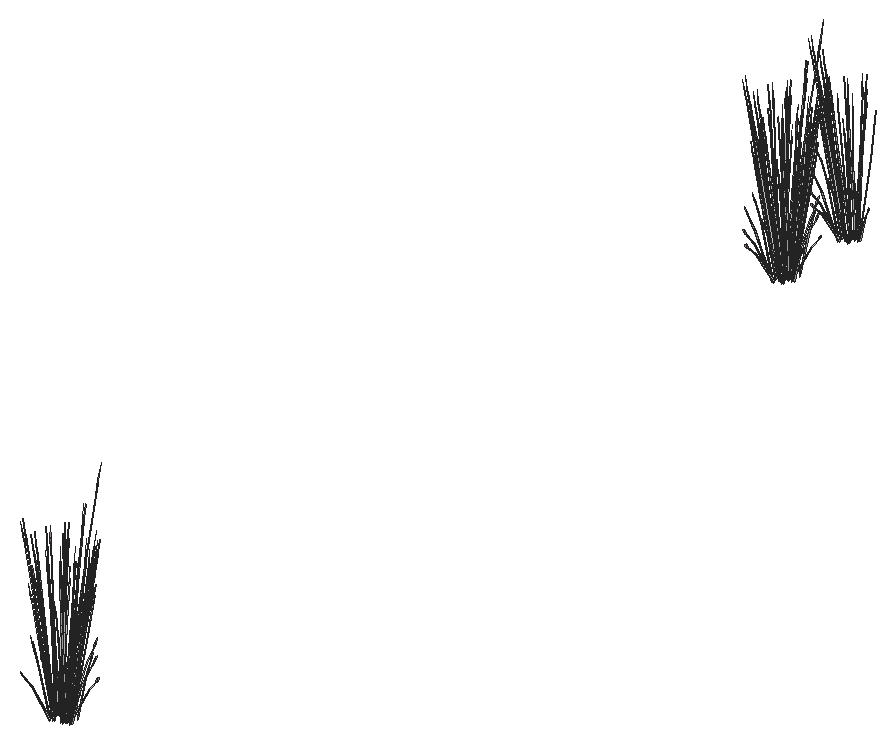
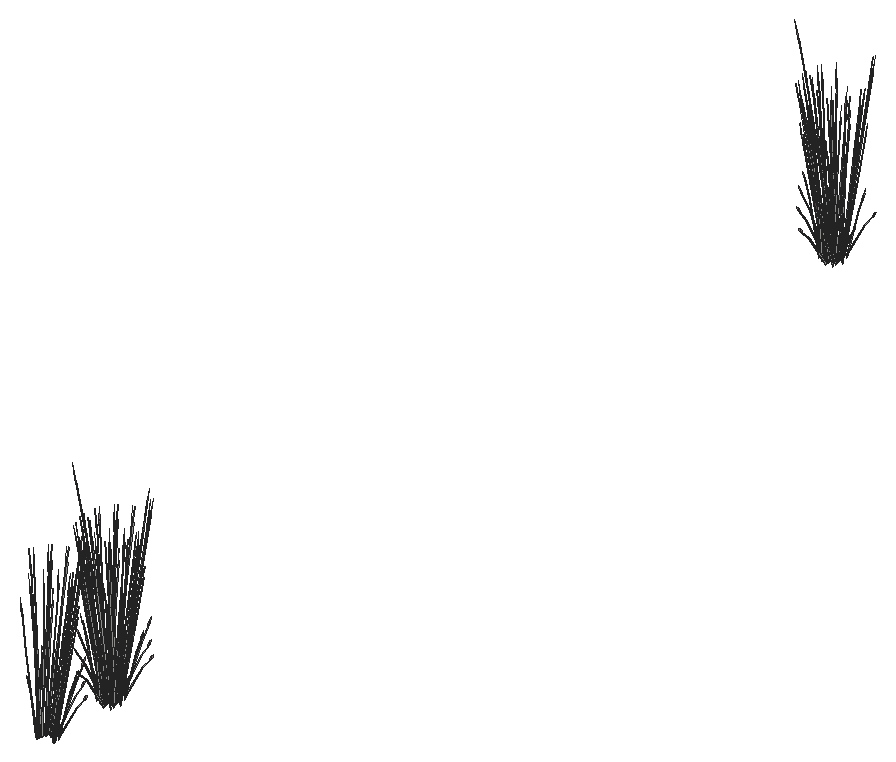
# SketchUp Ruby script. Lengths in inches.
U = 1.inch
M = Sketchup.active_model
def pt(a) = Geom::Point3d.new(a.map { |v| v * U })
def face(e, loops, mat)
  f = e.add_face(loops[0].map { |a| pt(a) })
  loops[1..].each { |l| e.add_face(l.map { |a| pt(a) }).erase! }
  f.material = f.back_material = mat if mat
  f
end
# faces: each face lists its corners as indices into pts; further lists are holes
def faces(e, pts, list, mat = nil) = list.each { |f| face(e, (f[0].is_a?(Array) ? f : [f]).map { |l| l.map { |i| pts[i] } }, mat) }
# xy, xz, yz: faces in a plane at the given z, y or x. An outline is a flat list of corners, or four numbers for a rectangle; further outlines are holes
def ring(l) = l.size == 4 ? [[l[0], l[1]], [l[2], l[1]], [l[2], l[3]], [l[0], l[3]]] : l.each_slice(2).to_a
def flat(e, list, mat, &to3) = list.each { |f| face(e, (f[0].is_a?(Array) ? f : [f]).map { |l| ring(l).map { |u, v| to3.(u, v) } }, mat) }
def xy(e, z, list, mat = nil) = flat(e, list, mat) { |x, y| [x, y, z] }
def xz(e, y, list, mat = nil) = flat(e, list, mat) { |x, z| [x, y, z] }
def yz(e, x, list, mat = nil) = flat(e, list, mat) { |y, z| [x, y, z] }
def lines(e, pts, list) = list.each { |a, b| e.add_line(pt(pts[a]), pt(pts[b])) }
# prism: a flat outline (further loops are holes) pulled along v
def prism(e, loops, v, mat = nil)
  f = face(e, loops, mat); d = Geom::Vector3d.new(v.map { |x| x * U })
  f.pushpull(f.normal.samedirection?(d) ? d.length : -d.length)
end
def box(e, o, s, mat = nil) = prism(e, [[o, [o[0] + s[0], o[1], o[2]], [o[0] + s[0], o[1] + s[1], o[2]], [o[0], o[1] + s[1], o[2]]]], [0, 0, s[2]], mat)
def at(x, y, z, deg = 0) = Geom::Transformation.translation(pt([x, y, z])) * Geom::Transformation.rotation(ORIGIN, Z_AXIS, deg.degrees)
def axes(o, x, y, z) = Geom::Transformation.new([*x, 0, *y, 0, *z, 0, *pt(o).to_a, 1])
def part(name) = M.definitions.add(name)
# library, detail: a bought-in or finely detailed component or shape, given as its bounding box
def library(name, o, s) = part(name).tap { |d| box(d.entities, o, s) }
def detail(e, o, s) = box(e.add_group.entities, o, s)
def put(e, d, t, mat = nil) = e.add_instance(d, t).tap { |i| i.material = mat if mat }
def group(e, t, mat = nil) = e.add_group.tap { |g| g.transformation = t; g.material = mat if mat }.entities
root = M.entities
M.materials.add("LightPink_Translucent").color = [144, 107, 117]
M.materials["LightPink_Translucent"].alpha = 0.75
c1 = part("blade")
p = [[2.15,0.21,22],[0,0.17,0],[0.09,0.45,0],[2.18,0.31,22],[2.29,0.31,22],[0.38,0.45,0],
  [2.48,0.24,33],[2.49,0.24,33],[2.48,0.22,33]]
faces(c1.entities,p,[[0,1,2,3],[4,5,2,3],[6,3,4,7],[8,0,3,6]])
c2 = part("seeds")
p = [[0.3,-0.1,1.38],[-0.01,-0.03,1.59],[-0.01,-0.03,0.03],[0.14,-0.07,-0.07],[0.29,-0.03,3],[0.15,0.01,3.11]]
faces(c2.entities,p,[[0,1,2,3],[1,0,4,5]],"LightPink_Translucent")
c3 = part("blade with seeds")
put(c3.entities,c1,at(0,0,0))
put(c3.entities,c2,axes([2.4,0.25,30.99],[1.5799,-0.05474,1.17369],[-0.12525,1.92788,0.29478],[-0.07173,-0.02425,1.56792]))
put(root,c3,axes([401.61,307.2,5.43],[-0.23555,0.44708,-0.13619],[-0.34112,-0.25757,-0.75594],[-0.11858,-0.12631,1.14864]))
put(root,c3,axes([403.22,307.69,4.73],[0.29004,0.02173,0.0643],[-0.00795,0.32812,0.50621],[0.03035,-0.12569,0.77189]))
put(root,c3,axes([403,307.91,5.05],[-0.23881,0.24554,0.35414],[-0.22606,-0.28036,-0.4572],[0.0344,-0.14245,0.87481]))
put(root,c3,axes([400.71,307.07,4.72],[-0.07594,-0.00329,1.74944],[-0.24177,0.32918,-0.27667],[-0.129,-0.06726,0.14031]))
put(root,c3,axes([403.58,308.71,5.03],[-0.32648,-0.25715,-0.1216],[0.18809,-0.3724,-0.67495],[0.09224,-0.12945,1.02557]))
put(root,c3,axes([401.59,307.57,5.05],[0.05451,0.37564,0.35414],[-0.31161,0.09919,-0.4572],[-0.0837,-0.10765,0.87481]))
put(root,c3,axes([400.65,307.8125,5.09],[0.29147,-0.34417,0.53763],[0.25138,0.3655,0.4433],[-0.13675,-0.06349,1.11249]))
put(root,c3,axes([404.38,308.6,4.71],[-0.0461,-0.00354,1.77383],[-0.19143,-0.37951,-0.16761],[0.07688,-0.12478,0.31391]))
put(root,c3,axes([400.78,307.8125,4.73],[0.01777,-0.35463,0.0643],[0.26836,0.00972,0.50621],[-0.1028,-0.03711,0.77189]))
put(root,c3,axes([403.42,308.67,5.05],[-0.30722,0.06665,0.35414],[-0.08112,-0.381,-0.4572],[0.08804,-0.10234,0.87481]))
put(root,c3,axes([403.7,308.61,4.73],[0.2423,0.19613,0.0643],[-0.14107,0.2793,0.50621],[0.07768,-0.0903,0.77189]))
put(root,c3,axes([403.63,308.53,4.73],[0.08753,0.42921,0.48003],[-0.34336,0.07449,0.3958],[0.1012,-0.10094,0.9933]))
put(root,c3,axes([404.55,309.05,4.72],[0.04898,-0.07104,1.74944],[-0.06269,-0.43574,-0.27667],[0.12289,-0.08262,0.14031]))
put(root,c3,axes([400.42,307.35,4.71],[0.02617,0.04654,1.77383],[-0.12614,0.41836,-0.16761],[-0.12775,0.00303,0.31391]))
put(root,c3,axes([400.97,308.08,5.05],[0.20082,0.29199,0.35414],[-0.2293,0.2764,-0.4572],[-0.1165,-0.04206,0.87481]))
put(root,c3,axes([400.91,307.89,5.03],[-0.0189,0.47427,-0.1216],[-0.35781,-0.01296,-0.67495],[-0.13781,-0.03295,1.02557]))
put(root,c3,axes([403.59,309.71,5.03],[-0.17758,-0.42229,-0.1216],[0.31518,-0.20752,-0.67495],[0.13282,-0.05572,1.02557]))
put(root,c3,axes([403.47,309.58,5.05],[-0.29332,-0.1301,0.35414],[0.08555,-0.37955,-0.4572],[0.11809,-0.0348,0.87481]))
put(root,c3,axes([400.4,308.89,4.73],[0.09971,-0.42522,0.48003],[0.32782,0.1454,0.3958],[-0.12892,0.02555,0.9933]))
put(root,c3,axes([400.37,308.78,4.73],[-0.12963,-0.31798,0.0643],[0.23638,-0.15564,0.50621],[-0.1042,0.03071,0.77189]))
put(root,c3,axes([403.73,309.7,4.73],[0.12963,0.31798,0.0643],[-0.23638,0.15564,0.50621],[0.1042,-0.03071,0.77189]))
put(root,c3,axes([403.71,309.59,4.73],[-0.09971,0.42522,0.48003],[-0.32782,-0.1454,0.3958],[0.12892,-0.02555,0.9933]))
put(root,c3,axes([400.64,308.9,5.05],[0.29332,0.1301,0.35414],[-0.08555,0.37955,-0.4572],[-0.11809,0.0348,0.87481]))
put(root,c3,axes([404.3,310.97,4.71],[-0.03191,-0.04083,1.77383],[0.06981,-0.43764,-0.16761],[0.12571,-0.02796,0.31391]))
put(root,c3,axes([400.14,309.19,4.72],[-0.05763,0.06055,1.74944],[0.0049,0.44239,-0.27667],[-0.13211,0.05753,0.14031]))
put(root,c3,axes([400.51,308.77,5.03],[0.17758,0.42229,-0.1216],[-0.31518,0.20752,-0.67495],[-0.13282,0.05572,1.02557]))
put(root,c3,axes([403.19,310.59,5.03],[0.0189,-0.47427,-0.1216],[0.35781,0.01296,-0.67495],[0.13781,0.03295,1.02557]))
put(root,c3,axes([403.14,310.4,5.05],[-0.20082,-0.29199,0.35414],[0.2293,-0.2764,-0.4572],[0.1165,0.04206,0.87481]))
put(root,c3,axes([403.5,310.3,4.72],[0.07571,-0.00789,1.74944],[0.20767,-0.36231,-0.27667],[0.13467,0.04783,0.14031]))
put(root,c3,axes([400.47,309.95,4.73],[-0.08753,-0.42921,0.48003],[0.34336,-0.07449,0.3958],[-0.1012,0.10094,0.9933]))
put(root,c3,axes([400.41,309.87,4.73],[-0.2423,-0.19613,0.0643],[0.14107,-0.2793,0.50621],[-0.07768,0.0903,0.77189]))
put(root,c3,axes([400.6875,309.81,5.05],[0.30722,-0.06665,0.35414],[0.08112,0.381,-0.4572],[-0.08804,0.10234,0.87481]))
put(root,c3,axes([399.5,309.64,4.71],[0.04504,0.01251,1.77383],[0.13934,0.41205,-0.16761],[-0.0922,0.10815,0.31391]))
put(root,c3,axes([403.32,310.67,4.73],[-0.01777,0.35463,0.0643],[-0.26836,-0.00972,0.50621],[0.1028,0.03711,0.77189]))
put(root,c3,axes([403.34,310.55,4.73],[-0.26024,0.30729,0.48003],[-0.22444,-0.32634,0.3958],[0.1221,0.05668,0.9933]))
put(root,c3,axes([399.99,310.89,5.65],[0.31145,0.12449,-0.06488],[-0.0958,0.38314,-0.29416],[-0.05094,0.05817,0.97024]))
put(root,c3,axes([402.52,310.91,5.05],[-0.05451,-0.37564,0.35414],[0.31161,-0.09919,-0.4572],[0.0837,0.10765,0.87481]))
put(root,c3,axes([402.72,308.75,4.47],[-0.30498,-0.24231,1.38283],[0.32203,-0.37727,0.59665],[0.0984,0.22736,1.33663]))
put(root,c3,axes([400.53,309.77,5.03],[0.32648,0.25715,-0.1216],[-0.18809,0.3724,-0.67495],[-0.09224,0.12945,1.02557]))
put(root,c3,axes([402.49,311.1,5.03],[0.21031,-0.39918,-0.1216],[0.30457,0.22997,-0.67495],[0.10587,0.11278,1.02557]))
put(root,c3,axes([401.1,310.57,5.05],[0.23881,-0.24554,0.35414],[0.22606,0.28036,-0.4572],[-0.0344,0.14245,0.87481]))
put(root,c3,axes([402.21,311.4375,4.71],[0.00104,-0.05646,1.77383],[0.30246,-0.2491,-0.16761],[0.10506,0.08891,0.31391]))
put(root,c3,axes([400.88,310.79,4.73],[-0.29004,-0.02173,0.0643],[0.00795,-0.32812,0.50621],[-0.03035,0.12569,0.77189]))
put(root,c3,axes([400.98,310.82,4.73],[-0.25132,-0.3182,0.48003],[0.2669,-0.27442,0.3958],[-0.04636,0.14929,0.9933]))
put(root,c3,axes([401.77,310.97,5.05],[0.1064,-0.35863,0.35414],[0.31043,0.1046,-0.4572],[0.02846,0.14439,0.87481]))
put(root,c3,axes([402.56,311.25,4.73],[-0.16041,0.29625,0.0643],[-0.22843,-0.17248,0.50621],[0.07385,0.09498,0.77189]))
put(root,c3,axes([402.1875,312.25,5.65],[0.2439,-0.26754,-0.06488],[0.22348,0.29302,-0.29416],[0.01573,0.08303,0.97024]))
put(root,c3,axes([402.63,311.17,4.73],[-0.35104,0.10702,0.48003],[-0.06092,-0.41983,0.3958],[0.08256,0.12373,0.9933]))
put(root,c3,axes([401.67,311.29,4.73],[-0.26007,0.1585,0.0643],[-0.12729,-0.28902,0.50621],[0.02512,0.1274,0.77189]))
put(root,c3,axes([400.15,310.84,4.72],[-0.00877,0.09229,1.74944],[0.24897,0.32105,-0.27667],[-0.06518,0.15182,0.14031]))
put(root,c3,axes([400.95,310.63,5.4],[0.3879,0.02311,-0.13498],[-0.0106,0.43749,-0.74919],[-0.02694,0.1685,1.13838]))
put(root,c3,axes([401.67,311.12,5.03],[0.34538,-0.21713,-0.1216],[0.16972,0.38536,-0.67495],[0.04557,0.16239,1.02557]))
put(root,c3,axes([401.77,311.26,5.0625],[-0.34777,-0.12192,0.53283],[0.11892,-0.40083,0.43934],[0.0209,0.15763,1.10256]))
put(root,c3,axes([400.125,311.79,4.71],[0.04004,-0.02816,1.77383],[0.33095,0.18728,-0.16761],[-0.00778,0.15594,0.31391]))
put(root,c3,axes([401.58,311.98,4.72],[0.04474,0.0751,1.74944],[0.36104,0.0295,-0.27667],[0.03631,0.16562,0.14031]))
put(root,c3,axes([401.89,516.79,4.72],[-0.05398,-0.06539,1.74944],[-0.36026,0.04145,-0.27667],[-0.0575,-0.15639,0.14031]))
put(root,c3,axes([403.51,517.59,4.72],[-0.00341,-0.09282,1.74944],[-0.28775,-0.26825,-0.27667],[0.04449,-0.16261,0.14031]))
put(root,c3,axes([403.43,517.25,4.71],[-0.03584,0.03562,1.77383],[-0.35118,-0.12018,-0.16761],[-0.01271,-0.15545,0.31391]))
put(root,c3,axes([401.52,516.57,4.71],[-0.00658,0.0559,1.77383],[-0.32474,0.20287,-0.16761],[-0.09556,-0.1037,0.31391]))
put(root,c3,axes([401.45,517.5625,5.09],[0.39316,-0.11987,0.53763],[0.06823,0.47021,0.4433],[-0.09247,-0.13858,1.11249]))
put(root,c3,axes([402.34,517.65,4.73],[0.34777,0.12192,0.48003],[-0.11892,0.40083,0.3958],[-0.0209,-0.15763,0.9933]))
put(root,c3,axes([402.4375,517.79,5.03],[-0.34538,0.21713,-0.1216],[-0.16972,-0.38536,-0.67495],[-0.04557,-0.16239,1.02557]))
put(root,c3,axes([403.15,518.28,5.03],[-0.3879,-0.02311,-0.1216],[0.0106,-0.43749,-0.67495],[0.02694,-0.1685,1.02557]))
put(root,c3,axes([402.43,517.62,4.73],[0.26007,-0.1585,0.0643],[0.12729,0.28902,0.50621],[-0.02512,-0.1274,0.77189]))
put(root,c3,axes([401.54,517.66,4.73],[0.16041,-0.29625,0.0643],[0.22843,0.17248,0.50621],[-0.07385,-0.09498,0.77189]))
put(root,c3,axes([402.33,517.95,5.05],[-0.1064,0.35863,0.35414],[-0.31043,-0.1046,-0.4572],[-0.02846,-0.14439,0.87481]))
put(root,c3,axes([403.125,518.1,4.73],[0.25132,0.3182,0.48003],[-0.2669,0.27442,0.3958],[0.04636,-0.14929,0.9933]))
put(root,c3,axes([401.61,517.63,5.43],[-0.23555,0.44708,-0.13619],[-0.34112,-0.25757,-0.75594],[-0.11858,-0.12631,1.14864]))
put(root,c3,axes([403.22,518.125,4.73],[0.29004,0.02173,0.0643],[-0.00795,0.32812,0.50621],[0.03035,-0.12569,0.77189]))
put(root,c3,axes([403,518.35,5.05],[-0.23881,0.24554,0.35414],[-0.22606,-0.28036,-0.4572],[0.0344,-0.14245,0.87481]))
put(root,c3,axes([400.71,517.51,4.72],[-0.07594,-0.00329,1.74944],[-0.24177,0.32918,-0.27667],[-0.129,-0.06726,0.14031]))
put(root,c3,axes([403.58,519.14,5.03],[-0.32648,-0.25715,-0.1216],[0.18809,-0.3724,-0.67495],[0.09224,-0.12945,1.02557]))
put(root,c3,axes([401.59,518.01,5.05],[0.05451,0.37564,0.35414],[-0.31161,0.09919,-0.4572],[-0.0837,-0.10765,0.87481]))
put(root,c3,axes([400.65,518.25,5.09],[0.29147,-0.34417,0.53763],[0.25138,0.3655,0.4433],[-0.13675,-0.06349,1.11249]))
put(root,c3,axes([404.38,519.03,4.71],[-0.0461,-0.00354,1.77383],[-0.19143,-0.37951,-0.16761],[0.07688,-0.12478,0.31391]))
put(root,c3,axes([400.78,518.25,4.73],[0.01777,-0.35463,0.0643],[0.26836,0.00972,0.50621],[-0.1028,-0.03711,0.77189]))
put(root,c3,axes([403.42,519.11,5.05],[-0.30722,0.06665,0.35414],[-0.08112,-0.381,-0.4572],[0.08804,-0.10234,0.87481]))
put(root,c3,axes([403.7,519.05,4.73],[0.2423,0.19613,0.0643],[-0.14107,0.2793,0.50621],[0.07768,-0.0903,0.77189]))
put(root,c3,axes([403.63,518.97,4.73],[0.08753,0.42921,0.48003],[-0.34336,0.07449,0.3958],[0.1012,-0.10094,0.9933]))
put(root,c3,axes([404.55,519.49,4.72],[0.04898,-0.07104,1.74944],[-0.06269,-0.43574,-0.27667],[0.12289,-0.08262,0.14031]))
put(root,c3,axes([400.42,517.78,4.71],[0.02617,0.04654,1.77383],[-0.12614,0.41836,-0.16761],[-0.12775,0.00303,0.31391]))
put(root,c3,axes([400.97,518.51,5.05],[0.20082,0.29199,0.35414],[-0.2293,0.2764,-0.4572],[-0.1165,-0.04206,0.87481]))
put(root,c3,axes([400.91,518.33,5.03],[-0.0189,0.47427,-0.1216],[-0.35781,-0.01296,-0.67495],[-0.13781,-0.03295,1.02557]))
put(root,c3,axes([403.59,520.15,5.03],[-0.17758,-0.42229,-0.1216],[0.31518,-0.20752,-0.67495],[0.13282,-0.05572,1.02557]))
put(root,c3,axes([403.47,520.02,5.05],[-0.29332,-0.1301,0.35414],[0.08555,-0.37955,-0.4572],[0.11809,-0.0348,0.87481]))
put(root,c3,axes([400.4,519.33,4.73],[0.09971,-0.42522,0.48003],[0.32782,0.1454,0.3958],[-0.12892,0.02555,0.9933]))
put(root,c3,axes([400.37,519.21,4.73],[-0.12963,-0.31798,0.0643],[0.23638,-0.15564,0.50621],[-0.1042,0.03071,0.77189]))
put(root,c3,axes([403.73,520.14,4.73],[0.12963,0.31798,0.0643],[-0.23638,0.15564,0.50621],[0.1042,-0.03071,0.77189]))
put(root,c3,axes([403.71,520.02,4.73],[-0.09971,0.42522,0.48003],[-0.32782,-0.1454,0.3958],[0.12892,-0.02555,0.9933]))
put(root,c3,axes([400.64,519.33,5.05],[0.29332,0.1301,0.35414],[-0.08555,0.37955,-0.4572],[-0.11809,0.0348,0.87481]))
put(root,c3,axes([404.3,521.4,4.71],[-0.03191,-0.04083,1.77383],[0.06981,-0.43764,-0.16761],[0.12571,-0.02796,0.31391]))
put(root,c3,axes([400.14,519.625,4.72],[-0.05763,0.06055,1.74944],[0.0049,0.44239,-0.27667],[-0.13211,0.05753,0.14031]))
put(root,c3,axes([400.51,519.2,5.03],[0.17758,0.42229,-0.1216],[-0.31518,0.20752,-0.67495],[-0.13282,0.05572,1.02557]))
put(root,c3,axes([403.19,521.02,5.03],[0.0189,-0.47427,-0.1216],[0.35781,0.01296,-0.67495],[0.13781,0.03295,1.02557]))
put(root,c3,axes([403.14,520.84,5.05],[-0.20082,-0.29199,0.35414],[0.2293,-0.2764,-0.4572],[0.1165,0.04206,0.87481]))
put(root,c3,axes([403.5,520.74,4.72],[0.07571,-0.00789,1.74944],[0.20767,-0.36231,-0.27667],[0.13467,0.04783,0.14031]))
put(root,c3,axes([400.47,520.39,4.73],[-0.08753,-0.42921,0.48003],[0.34336,-0.07449,0.3958],[-0.1012,0.10094,0.9933]))
put(root,c3,axes([400.41,520.3,4.73],[-0.2423,-0.19613,0.0643],[0.14107,-0.2793,0.50621],[-0.07768,0.0903,0.77189]))
put(root,c3,axes([400.6875,520.24,5.05],[0.30722,-0.06665,0.35414],[0.08112,0.381,-0.4572],[-0.08804,0.10234,0.87481]))
put(root,c3,axes([399.5,520.07,4.71],[0.04504,0.01251,1.77383],[0.13934,0.41205,-0.16761],[-0.0922,0.10815,0.31391]))
put(root,c3,axes([403.32,521.1,4.73],[-0.01777,0.35463,0.0643],[-0.26836,-0.00972,0.50621],[0.1028,0.03711,0.77189]))
put(root,c3,axes([403.34,520.99,4.73],[-0.26024,0.30729,0.48003],[-0.22444,-0.32634,0.3958],[0.1221,0.05668,0.9933]))
put(root,c3,axes([399.99,521.32,5.65],[0.31145,0.12449,-0.06488],[-0.0958,0.38314,-0.29416],[-0.05094,0.05817,0.97024]))
put(root,c3,axes([402.52,521.35,5.05],[-0.05451,-0.37564,0.35414],[0.31161,-0.09919,-0.4572],[0.0837,0.10765,0.87481]))
put(root,c3,axes([402.72,519.18,4.47],[-0.30498,-0.24231,1.38283],[0.32203,-0.37727,0.59665],[0.0984,0.22736,1.33663]))
put(root,c3,axes([400.53,520.21,5.03],[0.32648,0.25715,-0.1216],[-0.18809,0.3724,-0.67495],[-0.09224,0.12945,1.02557]))
put(root,c3,axes([402.49,521.54,5.03],[0.21031,-0.39918,-0.1216],[0.30457,0.22997,-0.67495],[0.10587,0.11278,1.02557]))
put(root,c3,axes([401.1,521,5.05],[0.23881,-0.24554,0.35414],[0.22606,0.28036,-0.4572],[-0.0344,0.14245,0.87481]))
put(root,c3,axes([402.21,521.87,4.71],[0.00104,-0.05646,1.77383],[0.30246,-0.2491,-0.16761],[0.10506,0.08891,0.31391]))
put(root,c3,axes([400.88,521.22,4.73],[-0.29004,-0.02173,0.0643],[0.00795,-0.32812,0.50621],[-0.03035,0.12569,0.77189]))
put(root,c3,axes([400.98,521.25,4.73],[-0.25132,-0.3182,0.48003],[0.2669,-0.27442,0.3958],[-0.04636,0.14929,0.9933]))
put(root,c3,axes([401.77,521.41,5.05],[0.1064,-0.35863,0.35414],[0.31043,0.1046,-0.4572],[0.02846,0.14439,0.87481]))
put(root,c3,axes([402.56,521.6875,4.73],[-0.16041,0.29625,0.0643],[-0.22843,-0.17248,0.50621],[0.07385,0.09498,0.77189]))
put(root,c3,axes([402.1875,522.68,5.65],[0.2439,-0.26754,-0.06488],[0.22348,0.29302,-0.29416],[0.01573,0.08303,0.97024]))
put(root,c3,axes([402.63,521.6,4.73],[-0.35104,0.10702,0.48003],[-0.06092,-0.41983,0.3958],[0.08256,0.12373,0.9933]))
put(root,c3,axes([401.67,521.73,4.73],[-0.26007,0.1585,0.0643],[-0.12729,-0.28902,0.50621],[0.02512,0.1274,0.77189]))
put(root,c3,axes([400.15,521.28,4.72],[-0.00877,0.09229,1.74944],[0.24897,0.32105,-0.27667],[-0.06518,0.15182,0.14031]))
put(root,c3,axes([400.95,521.07,5.4],[0.3879,0.02311,-0.13498],[-0.0106,0.43749,-0.74919],[-0.02694,0.1685,1.13838]))
put(root,c3,axes([401.67,521.56,5.03],[0.34538,-0.21713,-0.1216],[0.16972,0.38536,-0.67495],[0.04557,0.16239,1.02557]))
put(root,c3,axes([401.77,521.7,5.0625],[-0.34777,-0.12192,0.53283],[0.11892,-0.40083,0.43934],[0.0209,0.15763,1.10256]))
put(root,c3,axes([400.125,522.22,4.71],[0.04004,-0.02816,1.77383],[0.33095,0.18728,-0.16761],[-0.00778,0.15594,0.31391]))
put(root,c3,axes([401.58,522.42,4.72],[0.04474,0.0751,1.74944],[0.36104,0.0295,-0.27667],[0.03631,0.16562,0.14031]))
put(root,c3,axes([401.89,536.01,4.72],[-0.05398,-0.06539,1.74944],[-0.36026,0.04145,-0.27667],[-0.0575,-0.15639,0.14031]))
put(root,c3,axes([403.51,536.82,4.72],[-0.00341,-0.09282,1.74944],[-0.28775,-0.26825,-0.27667],[0.04449,-0.16261,0.14031]))
put(root,c3,axes([403.43,536.48,4.71],[-0.03584,0.03562,1.77383],[-0.35118,-0.12018,-0.16761],[-0.01271,-0.15545,0.31391]))
put(root,c3,axes([401.52,535.8,4.71],[-0.00658,0.0559,1.77383],[-0.32474,0.20287,-0.16761],[-0.09556,-0.1037,0.31391]))
put(root,c3,axes([401.45,536.79,5.09],[0.39316,-0.11987,0.53763],[0.06823,0.47021,0.4433],[-0.09247,-0.13858,1.11249]))
put(root,c3,axes([402.34,536.88,4.73],[0.34777,0.12192,0.48003],[-0.11892,0.40083,0.3958],[-0.0209,-0.15763,0.9933]))
put(root,c3,axes([402.4375,537.02,5.03],[-0.34538,0.21713,-0.1216],[-0.16972,-0.38536,-0.67495],[-0.04557,-0.16239,1.02557]))
put(root,c3,axes([403.15,537.51,5.03],[-0.3879,-0.02311,-0.1216],[0.0106,-0.43749,-0.67495],[0.02694,-0.1685,1.02557]))
put(root,c3,axes([402.43,536.85,4.73],[0.26007,-0.1585,0.0643],[0.12729,0.28902,0.50621],[-0.02512,-0.1274,0.77189]))
put(root,c3,axes([401.54,536.89,4.73],[0.16041,-0.29625,0.0643],[0.22843,0.17248,0.50621],[-0.07385,-0.09498,0.77189]))
put(root,c3,axes([402.33,537.17,5.05],[-0.1064,0.35863,0.35414],[-0.31043,-0.1046,-0.4572],[-0.02846,-0.14439,0.87481]))
put(root,c3,axes([403.125,537.33,4.73],[0.25132,0.3182,0.48003],[-0.2669,0.27442,0.3958],[0.04636,-0.14929,0.9933]))
put(root,c3,axes([401.61,536.86,5.43],[-0.23555,0.44708,-0.13619],[-0.34112,-0.25757,-0.75594],[-0.11858,-0.12631,1.14864]))
put(root,c3,axes([403.22,537.36,4.73],[0.29004,0.02173,0.0643],[-0.00795,0.32812,0.50621],[0.03035,-0.12569,0.77189]))
put(root,c3,axes([403,537.58,5.05],[-0.23881,0.24554,0.35414],[-0.22606,-0.28036,-0.4572],[0.0344,-0.14245,0.87481]))
put(root,c3,axes([400.71,536.73,4.72],[-0.07594,-0.00329,1.74944],[-0.24177,0.32918,-0.27667],[-0.129,-0.06726,0.14031]))
put(root,c3,axes([403.58,538.37,5.03],[-0.32648,-0.25715,-0.1216],[0.18809,-0.3724,-0.67495],[0.09224,-0.12945,1.02557]))
put(root,c3,axes([401.59,537.23,5.05],[0.05451,0.37564,0.35414],[-0.31161,0.09919,-0.4572],[-0.0837,-0.10765,0.87481]))
put(root,c3,axes([400.65,537.48,5.09],[0.29147,-0.34417,0.53763],[0.25138,0.3655,0.4433],[-0.13675,-0.06349,1.11249]))
put(root,c3,axes([404.38,538.26,4.71],[-0.0461,-0.00354,1.77383],[-0.19143,-0.37951,-0.16761],[0.07688,-0.12478,0.31391]))
put(root,c3,axes([400.78,537.48,4.73],[0.01777,-0.35463,0.0643],[0.26836,0.00972,0.50621],[-0.1028,-0.03711,0.77189]))
put(root,c3,axes([403.42,538.34,5.05],[-0.30722,0.06665,0.35414],[-0.08112,-0.381,-0.4572],[0.08804,-0.10234,0.87481]))
put(root,c3,axes([403.7,538.28,4.73],[0.2423,0.19613,0.0643],[-0.14107,0.2793,0.50621],[0.07768,-0.0903,0.77189]))
put(root,c3,axes([403.63,538.19,4.73],[0.08753,0.42921,0.48003],[-0.34336,0.07449,0.3958],[0.1012,-0.10094,0.9933]))
put(root,c3,axes([404.55,538.71,4.72],[0.04898,-0.07104,1.74944],[-0.06269,-0.43574,-0.27667],[0.12289,-0.08262,0.14031]))
put(root,c3,axes([400.42,537.01,4.71],[0.02617,0.04654,1.77383],[-0.12614,0.41836,-0.16761],[-0.12775,0.00303,0.31391]))
put(root,c3,axes([400.97,537.74,5.05],[0.20082,0.29199,0.35414],[-0.2293,0.2764,-0.4572],[-0.1165,-0.04206,0.87481]))
put(root,c3,axes([400.91,537.55,5.03],[-0.0189,0.47427,-0.1216],[-0.35781,-0.01296,-0.67495],[-0.13781,-0.03295,1.02557]))
put(root,c3,axes([403.59,539.375,5.03],[-0.17758,-0.42229,-0.1216],[0.31518,-0.20752,-0.67495],[0.13282,-0.05572,1.02557]))
put(root,c3,axes([403.47,539.25,5.05],[-0.29332,-0.1301,0.35414],[0.08555,-0.37955,-0.4572],[0.11809,-0.0348,0.87481]))
put(root,c3,axes([400.4,538.55,4.73],[0.09971,-0.42522,0.48003],[0.32782,0.1454,0.3958],[-0.12892,0.02555,0.9933]))
put(root,c3,axes([400.37,538.44,4.73],[-0.12963,-0.31798,0.0643],[0.23638,-0.15564,0.50621],[-0.1042,0.03071,0.77189]))
put(root,c3,axes([403.73,539.37,4.73],[0.12963,0.31798,0.0643],[-0.23638,0.15564,0.50621],[0.1042,-0.03071,0.77189]))
